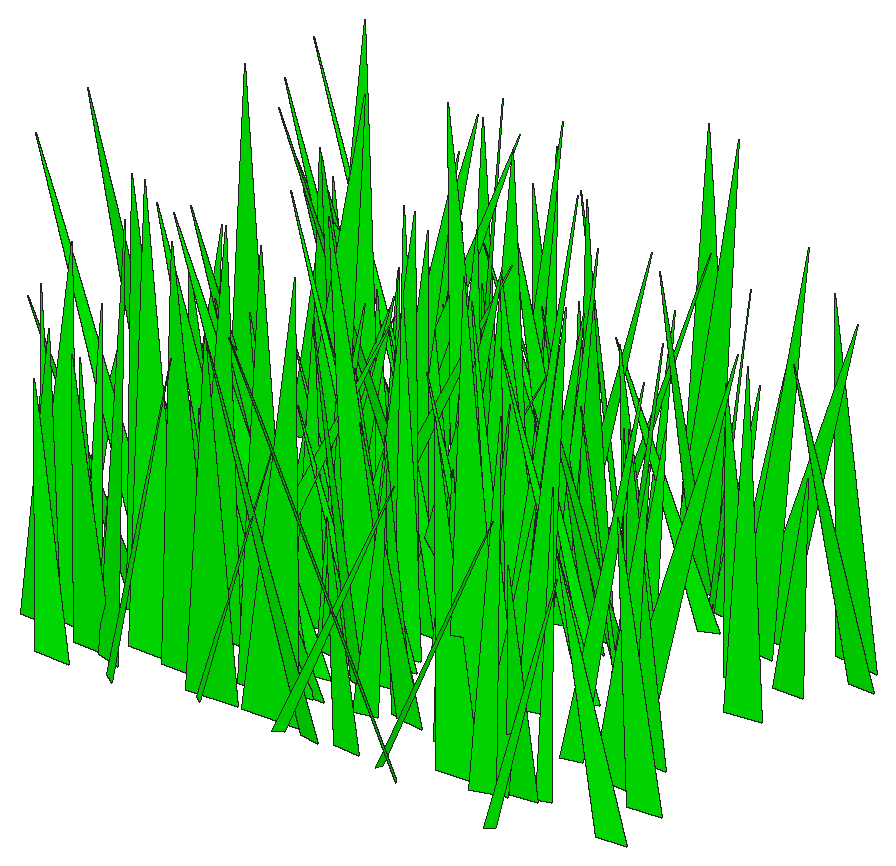
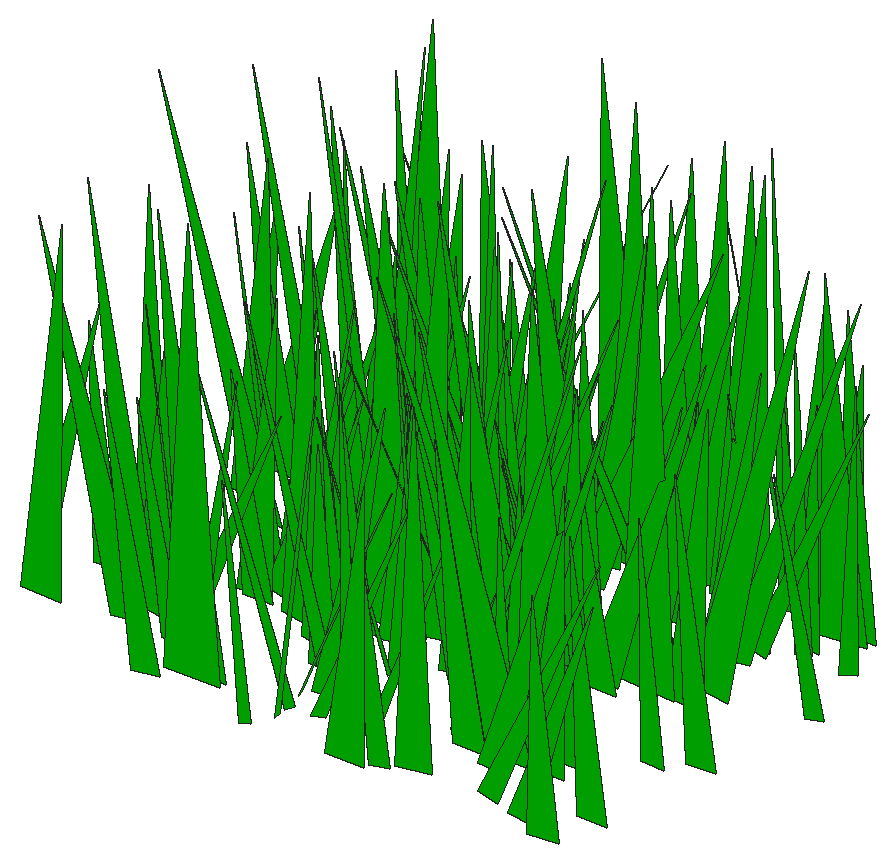
# SketchUp Ruby script. Lengths in inches.
U = 1.inch
M = Sketchup.active_model
def pt(a) = Geom::Point3d.new(a.map { |v| v * U })
def face(e, loops, mat)
  f = e.add_face(loops[0].map { |a| pt(a) })
  loops[1..].each { |l| e.add_face(l.map { |a| pt(a) }).erase! }
  f.material = f.back_material = mat if mat
  f
end
# faces: each face lists its corners as indices into pts; further lists are holes
def faces(e, pts, list, mat = nil) = list.each { |f| face(e, (f[0].is_a?(Array) ? f : [f]).map { |l| l.map { |i| pts[i] } }, mat) }
# xy, xz, yz: faces in a plane at the given z, y or x. An outline is a flat list of corners, or four numbers for a rectangle; further outlines are holes
def ring(l) = l.size == 4 ? [[l[0], l[1]], [l[2], l[1]], [l[2], l[3]], [l[0], l[3]]] : l.each_slice(2).to_a
def flat(e, list, mat, &to3) = list.each { |f| face(e, (f[0].is_a?(Array) ? f : [f]).map { |l| ring(l).map { |u, v| to3.(u, v) } }, mat) }
def xy(e, z, list, mat = nil) = flat(e, list, mat) { |x, y| [x, y, z] }
def xz(e, y, list, mat = nil) = flat(e, list, mat) { |x, z| [x, y, z] }
def yz(e, x, list, mat = nil) = flat(e, list, mat) { |y, z| [x, y, z] }
def lines(e, pts, list) = list.each { |a, b| e.add_line(pt(pts[a]), pt(pts[b])) }
# prism: a flat outline (further loops are holes) pulled along v
def prism(e, loops, v, mat = nil)
  f = face(e, loops, mat); d = Geom::Vector3d.new(v.map { |x| x * U })
  f.pushpull(f.normal.samedirection?(d) ? d.length : -d.length)
end
def box(e, o, s, mat = nil) = prism(e, [[o, [o[0] + s[0], o[1], o[2]], [o[0] + s[0], o[1] + s[1], o[2]], [o[0], o[1] + s[1], o[2]]]], [0, 0, s[2]], mat)
def at(x, y, z, deg = 0) = Geom::Transformation.translation(pt([x, y, z])) * Geom::Transformation.rotation(ORIGIN, Z_AXIS, deg.degrees)
def axes(o, x, y, z) = Geom::Transformation.new([*x, 0, *y, 0, *z, 0, *pt(o).to_a, 1])
def part(name) = M.definitions.add(name)
# library, detail: a bought-in or finely detailed component or shape, given as its bounding box
def library(name, o, s) = part(name).tap { |d| box(d.entities, o, s) }
def detail(e, o, s) = box(e.add_group.entities, o, s)
def put(e, d, t, mat = nil) = e.add_instance(d, t).tap { |i| i.material = mat if mat }
def group(e, t, mat = nil) = e.add_group.tap { |g| g.transformation = t; g.material = mat if mat }.entities
root = M.entities
M.materials.add("[0065_Lime]").color = [0, 255, 0]
c1 = part("fur_instance\#9")
p = [[0.8125,0,1.79],[0.67,-0.02,1.48],[0,-0.11,0],[0,0.11,0]]
faces(c1.entities,p,[[0,1,2,3]])
put(root,c1,axes([47.23,21.45,1.48],[4.4292,-0.25222,2.09729],[2.23078,0.69345,-0.32267],[-2.2121,0.1943,3.87394]),"[0065_Lime]")
put(root,c1,axes([46.43,23.84,1.48],[3.37907,-0.32218,0.93432],[2.44204,0.48577,-0.23052],[-0.78289,0.12464,3.31359]),"[0065_Lime]")
put(root,c1,axes([47.11,27.62,1.48],[2.95,-0.56759,1.1379],[4.20157,0.42898,-0.03681],[-0.78709,0.16263,4.06838]),"[0065_Lime]")
put(root,c1,axes([49.87,22.73,1.48],[-7.12168,0.44148,0.88746],[-3.20755,-1.0075,-0.23593],[0.8793,-0.09949,6.32715]),"[0065_Lime]")
put(root,c1,axes([49.4,24.42,1.48],[-5.61424,-0.877,1.17279],[6.33943,-0.79934,0.04951],[0.91831,0.15643,6.82825]),"[0065_Lime]")
put(root,c1,axes([49.0625,32.54,1.48],[-2.29448,-0.55155,0.20796],[3.93163,-0.32033,0.23303],[-0.11894,0.0513,3.69087]),"[0065_Lime]")
put(root,c1,axes([48,32.97,1.48],[-0.85767,0.65446,0.46875],[-4.67473,-0.1264,0.25449],[0.4141,-0.07144,3.84377]),"[0065_Lime]")
put(root,c1,axes([49.78,22,1.48],[-4.29564,-0.46868,0.1591],[3.34086,-0.60308,0.15104],[0.04046,0.03747,4.42116]),"[0065_Lime]")
put(root,c1,axes([47.57,31.5,1.48],[2.89563,-0.58713,0.52134],[4.16251,0.41505,0.36618],[-0.73658,0.03742,4.11881]),"[0065_Lime]")
put(root,c1,axes([48.19,28.26,1.48],[-2.15247,-0.46889,1.6236],[3.6972,-0.34608,-0.10604],[1.204,0.22446,3.22823]),"[0065_Lime]")
put(root,c1,axes([48.4,20.17,1.48],[-1.17696,0.95171,1.12358],[-6.87953,-0.18043,0.35304],[0.67218,-0.1802,5.58054]),"[0065_Lime]")
put(root,c1,axes([48.27,19.83,1.48],[0.67146,-0.84255,0.3532],[6.0109,0.09305,-0.12296],[0.10231,0.06299,4.90622]),"[0065_Lime]")
put(root,c1,axes([50.43,32.16,1.48],[-4.06579,-0.47447,0.17632],[3.38281,-0.56903,0.30067],[-0.07001,0.0594,4.28842]),"[0065_Lime]")
put(root,c1,axes([48.91,21.03,1.48],[-2.22554,-0.48819,1.56603],[3.88886,-0.33093,0.19972],[0.80849,0.24793,3.35014]),"[0065_Lime]")
put(root,c1,axes([48.77,21.35,1.48],[4.78206,-0.26753,1.75717],[2.0609,0.72896,0.00803],[-2.01098,0.11088,4.18673]),"[0065_Lime]")
put(root,c1,axes([49.67,18.54,1.48],[-1.89741,0.6773,0.01247],[-4.81189,-0.2663,0.24042],[0.28063,0.01321,4.20666]),"[0065_Lime]")
put(root,c1,axes([49.51,25.29,1.48],[-0.06571,-0.77818,0.68187],[5.59689,-0.00459,0.18134],[-0.21553,0.11807,4.50131]),"[0065_Lime]")
put(root,c1,axes([49.87,23.66,1.48],[-2.57835,-0.75231,0.50608],[5.36351,-0.3677,-0.23597],[0.53244,0.06089,4.82782]),"[0065_Lime]")
put(root,c1,axes([50.07,30.28,1.48],[-1.31314,0.71883,1.28918],[-5.35298,-0.18318,-0.18498],[0.16371,-0.22381,4.29201]),"[0065_Lime]")
put(root,c1,axes([51.72,29.89,1.48],[-6.71262,0.39548,0.95592],[-2.87689,-0.95358,-0.14683],[1.01275,-0.08753,5.91881]),"[0065_Lime]")
put(root,c1,axes([49.99,29.61,1.48],[-0.14768,-1.00225,0.25056],[7.13724,-0.02175,-0.13172],[0.16842,0.04279,5.80148]),"[0065_Lime]")
put(root,c1,axes([50.23,19.51,1.48],[-0.42754,-0.82229,0.31765],[5.8646,-0.06048,-0.02331],[0.0571,0.05443,4.77261]),"[0065_Lime]")
put(root,c1,axes([51.22,30.94,1.48],[-2.63269,-0.7093,0.04104],[5.0473,-0.37,-0.05484],[0.08311,0.0019,4.63047]),"[0065_Lime]")
put(root,c1,axes([50.49,21.79,1.48],[0.80245,-1.23017,0.66425],[8.78031,0.11819,0.31677],[-0.46395,0.10914,7.1439]),"[0065_Lime]")
put(root,c1,axes([51.98,25.59,1.48],[-4.04821,-0.74608,0.44801],[5.33652,-0.56795,0.21143],[0.12629,0.08372,5.42684]),"[0065_Lime]")
put(root,c1,axes([50.375,19.72,1.48],[3.47743,-0.24304,1.39652],[2.02024,0.52259,-0.28083],[-1.36303,0.15451,3.14665]),"[0065_Lime]")
put(root,c1,axes([50.79,25.26,1.48],[-2.93002,-1.1104,3.08242],[8.67927,-0.44549,0.08108],[1.21487,0.50458,6.85493]),"[0065_Lime]")
put(root,c1,axes([50.83,29.24,1.48],[-0.74135,1.30052,0.49003],[-9.27229,-0.1059,0.13632],[0.21549,-0.08248,7.55119]),"[0065_Lime]")
put(root,c1,axes([50.4,21.22,1.48],[2.7644,0.47656,0.67631],[-3.38313,0.40243,-0.35262],[-0.86477,-0.05094,3.54148]),"[0065_Lime]")
put(root,c1,axes([52.57,22.97,1.48],[-5.0713,0.71122,0.87309],[-5.15149,-0.71375,-0.31492],[0.48207,-0.14533,5.81953]),"[0065_Lime]")
put(root,c1,axes([51.93,24.83,1.48],[-1.94658,-0.68112,0.62782],[4.90798,-0.26876,0.29807],[-0.05682,0.11979,4.23839]),"[0065_Lime]")
put(root,c1,axes([50.88,19.33,1.48],[-6.55389,-0.45489,2.97592],[3.6482,-1.02785,0.05119],[3.24894,0.23653,5.94567]),"[0065_Lime]")
put(root,c1,axes([53.26,29.8125,1.48],[-8.14536,0.22202,1.03626],[-1.53362,-1.15823,0.33952],[1.32949,0.02421,6.7405]),"[0065_Lime]")
put(root,c1,axes([51.75,20.25,1.48],[-2.01765,1.17085,1.09515],[-8.43103,-0.28877,0.06798],[0.39907,-0.18107,6.97322]),"[0065_Lime]")
put(root,c1,axes([50.26,28.41,1.48],[3.82268,0.39815,0.44658],[-2.87134,0.53759,0.20153],[-0.29195,-0.07403,3.8652]),"[0065_Lime]")
put(root,c1,axes([51.46,30.24,1.48],[-2.79502,0.37495,1.5795],[-3.00222,-0.43736,-0.03599],[1.37024,-0.19344,3.14302]),"[0065_Lime]")
put(root,c1,axes([52.24,27.98,1.48],[-1.87166,-1.01335,0.70925],[7.25339,-0.26757,-0.14548],[0.39328,0.1122,6.05855]),"[0065_Lime]")
put(root,c1,axes([52.27,21.88,1.48],[3.18095,-0.24835,1.55497],[1.95904,0.50766,0.06543],[-1.71476,0.11928,2.95928]),"[0065_Lime]")
put(root,c1,axes([54.47,28.02,1.48],[-7.29785,-0.48829,0.51769],[3.46077,-1.02937,-0.2554],[0.7096,-0.00154,6.56981]),"[0065_Lime]")
put(root,c1,axes([51.38,28.3125,1.48],[-2.54827,-0.40995,2.16007],[3.3881,-0.45499,-0.24896],[2.02097,0.24586,3.14103]),"[0065_Lime]")
put(root,c1,axes([51.65,27.09,1.48],[3.53407,0.45813,0.7792],[-3.26627,0.51155,-0.27665],[-0.93747,-0.05523,3.90131]),"[0065_Lime]")
put(root,c1,axes([52.64,28.46,1.48],[3.40763,-0.27593,1.90182],[2.47601,0.5378,-0.32072],[-1.78658,0.21906,3.18296]),"[0065_Lime]")
put(root,c1,axes([51.17,30.375,1.48],[3.15132,0.98904,0.84715],[-7.11513,0.4384,0.36136],[-0.01573,-0.15909,6.26244]),"[0065_Lime]")
put(root,c1,axes([52.25,22.07,1.48],[1.96154,0.9156,2.8317],[-7.35658,0.28841,0.24682],[-0.67613,-0.48175,5.52958]),"[0065_Lime]")
put(root,c1,axes([51.5,18.59,1.48],[5.99318,0.19121,1.37292],[-1.45464,0.87161,0.13377],[-1.60761,-0.07586,4.99721]),"[0065_Lime]")
put(root,c1,axes([52.79,32.27,1.48],[-4.08034,0.68378,1.87075],[-5.08436,-0.62274,0.28991],[1.76586,-0.21302,5.15743]),"[0065_Lime]")
put(root,c1,axes([52.1,26.04,1.48],[2.00461,1.23257,1.45558],[-8.95105,0.28033,0.2018],[-0.15193,-0.25296,7.31616]),"[0065_Lime]")
put(root,c1,axes([52.97,20.05,1.48],[-0.12204,-1.13464,1.32187],[8.23646,-0.0155,0.05733],[-0.04733,0.22847,6.56856]),"[0065_Lime]")
put(root,c1,axes([52.37,30.51,1.48],[1.80119,0.69196,1.38518],[-5.20498,0.25057,0.28386],[-0.23909,-0.24194,4.2556]),"[0065_Lime]")
put(root,c1,axes([55.44,21.94,1.48],[-6.13954,0.70094,0.10061],[-4.98964,-0.86263,-0.07578],[0.03724,-0.02112,6.43408]),"[0065_Lime]")
put(root,c1,axes([54.4,25.27,1.48],[-4.60606,0.01384,0.73954],[-0.16863,-0.65763,-0.2825],[0.89882,-0.05246,3.73682]),"[0065_Lime]")
put(root,c1,axes([51.26,29.71,1.48],[6.63129,0.66177,0.71913],[-4.76645,0.93275,0.31877],[-0.49172,-0.11701,6.60818]),"[0065_Lime]")
put(root,c1,axes([53.15,31.33,1.48],[7.30412,-0.01994,2.19479],[0.0411,1.09352,0.24234],[-2.70166,-0.03726,5.93745]),"[0065_Lime]")
put(root,c1,axes([53.78,23.91,1.48],[3.70468,-0.58018,1.44831],[4.23681,0.55898,0.33298],[-1.50587,0.14537,4.49994]),"[0065_Lime]")
put(root,c1,axes([54.49,32.97,1.48],[-1.3105,0.78874,0.29597],[-5.6249,-0.18366,-0.07831],[-0.01122,-0.05287,4.68793]),"[0065_Lime]")
put(root,c1,axes([55.26,30.56,1.48],[-3.69418,-0.23516,0.4105],[1.71348,-0.51995,0.22151],[0.34542,0.06432,3.2914]),"[0065_Lime]")
put(root,c1,axes([53.58,32.66,1.48],[6.56596,-0.3231,1.71503],[2.333,0.96687,0.19409],[-2.07118,0.0648,5.65553]),"[0065_Lime]")
put(root,c1,axes([54.17,19.44,1.48],[1.31811,-1.07028,0.00043],[7.60972,0.18505,0.26911],[-0.32609,-0.00785,6.28185]),"[0065_Lime]")
put(root,c1,axes([53.68,25.57,1.48],[2.35032,0.47932,0.58753],[-3.48355,0.32803,0.25266],[-0.14903,-0.10848,3.36001]),"[0065_Lime]")
put(root,c1,axes([53.28,27.46,1.48],[6.49266,-0.71764,1.52624],[5.25924,0.93295,-0.10336],[-1.39403,0.17738,6.71846]),"[0065_Lime]")
put(root,c1,axes([54.53,32.6,1.48],[5.73438,-0.26141,2.21074],[2.2169,0.87344,-0.3438],[-2.43578,0.17953,4.89168]),"[0065_Lime]")
put(root,c1,axes([52.2,22.8,1.48],[6.30052,0.49234,0.17348],[-3.50968,0.88467,0.20459],[-0.06398,-0.04546,5.86051]),"[0065_Lime]")
put(root,c1,axes([55.14,27.64,1.48],[-4.02548,0.57884,1.30914],[-4.18319,-0.59759,0.34327],[1.43523,-0.11828,4.67236]),"[0065_Lime]")
put(root,c1,axes([56.44,31.6,1.48],[-4.74214,0.23885,0.25626],[-1.69737,-0.66782,0.07541],[0.32786,-0.00265,4.09694]),"[0065_Lime]")
put(root,c1,axes([55.69,20.93,1.48],[-4.58117,0.66209,1.03081],[-4.75356,-0.66072,0.24269],[1.10036,-0.09778,5.34006]),"[0065_Lime]")
put(root,c1,axes([54.57,26.84,1.48],[0.12519,0.90816,1.54224],[-6.73073,0.00704,0.22252],[0.24835,-0.26691,5.25331]),"[0065_Lime]")
put(root,c1,axes([55.18,24.41,1.48],[-3.13246,0.48304,0.9905],[-3.46535,-0.46453,0.33998],[1.13621,-0.08507,3.76765]),"[0065_Lime]")
put(root,c1,axes([54.83,23.56,1.48],[2.42727,-0.58743,1.01618],[4.27025,0.36107,0.24531],[-0.89544,0.12954,3.9244]),"[0065_Lime]")
put(root,c1,axes([56.2,21.03,1.48],[-2.4252,-0.49908,0.18297],[3.55594,-0.33828,0.26587],[-0.14382,0.05196,3.48816]),"[0065_Lime]")
put(root,c1,axes([53.95,19.16,1.48],[5.0056,0.1335,0.79462],[-0.96794,0.71617,0.00241],[-0.9592,-0.02601,4.14431]),"[0065_Lime]")
put(root,c1,axes([55.13,20.45,1.48],[-0.75065,-1.13661,1.87157],[8.39979,-0.11704,-0.15281],[0.40697,0.31931,6.606]),"[0065_Lime]")
put(root,c1,axes([56.58,22.91,1.48],[-4.12783,0.24962,0.61548],[-1.85509,-0.58231,-0.31794],[0.53571,-0.09303,3.64151]),"[0065_Lime]")
put(root,c1,axes([54.625,28.02,1.48],[3.10545,0.5802,0.72513],[-4.18816,0.44317,-0.01474],[-0.55054,-0.09856,4.20248]),"[0065_Lime]")
put(root,c1,axes([55.38,23.04,1.48],[-1.76012,-0.65762,1.78715],[5.0861,-0.27878,-0.12322],[0.92795,0.28065,4.06522]),"[0065_Lime]")
put(root,c1,axes([57.03,23.62,1.48],[-4.37671,0.58013,0.55057],[-4.16274,-0.61761,-0.08801],[0.41758,-0.07638,4.89324]),"[0065_Lime]")
put(root,c1,axes([57.63,23.08,1.48],[-8.16969,0.19733,1.17611],[-1.34853,-1.16551,0.35474],[1.49801,0.02694,6.73345]),"[0065_Lime]")
put(root,c1,axes([57.46,19.31,1.48],[-5.96996,-0.449,0.97046],[3.29159,-0.84699,0.26596],[0.89398,0.12015,5.50145]),"[0065_Lime]")
put(root,c1,axes([56.87,30.63,1.48],[-3.63253,0.64668,0.93106],[-4.7153,-0.51413,-0.20621],[0.50577,-0.14862,4.76459]),"[0065_Lime]")
put(root,c1,axes([53.13,26.32,1.48],[7.25901,-0.32559,0.26107],[2.32884,1.01973,-0.22824],[-0.22015,0.0513,6.19388]),"[0065_Lime]")
put(root,c1,axes([56.66,22.29,1.48],[-5.5855,-0.37084,1.47546],[2.64957,-0.82297,-0.29467],[1.79854,0.06073,5.01627]),"[0065_Lime]")
put(root,c1,axes([57.53,30.96,1.48],[-4.58838,-0.01997,0.33202],[0.1625,-0.64643,0.18288],[0.4005,0.03348,3.72956]),"[0065_Lime]")
put(root,c1,axes([56.16,28.53,1.48],[-3.20737,-0.60107,1.34124],[4.39299,-0.48382,-0.31489],[1.31071,0.15074,4.33747]),"[0065_Lime]")
put(root,c1,axes([55.98,24.45,1.48],[-6.19842,0.14888,2.41809],[-1.09563,-0.96491,0.13257],[2.95966,-0.04539,5.11329]),"[0065_Lime]")
put(root,c1,axes([57.03,22.62,1.48],[-3.80468,0.96953,1.86173],[-7.23157,-0.54178,-0.32383],[0.74076,-0.30941,6.40083]),"[0065_Lime]")
put(root,c1,axes([57.16,25.25,1.48],[-4.92857,0.27745,1.14097],[-2.10496,-0.71174,-0.21653],[1.19806,-0.10912,4.31329]),"[0065_Lime]")
put(root,c1,axes([57.02,26.66,1.48],[-6.50986,0.84997,2.24696],[-6.23212,-0.9693,0.34024],[2.31956,-0.21884,7.22025]),"[0065_Lime]")
put(root,c1,axes([56.01,19.54,1.48],[2.78966,-1.11729,1.54568],[8.15235,0.40126,-0.01582],[-0.61028,0.25289,6.85414]),"[0065_Lime]")
put(root,c1,axes([57.28,32.21,1.48],[-5.8952,0.0148,1.57894],[-0.00586,-0.87111,0.25906],[1.94397,0.04224,4.789]),"[0065_Lime]")
put(root,c1,axes([56.15,24.26,1.48],[0.8068,-1.11162,2.12559],[8.32936,0.09956,-0.34711],[0.18211,0.37118,6.45891]),"[0065_Lime]")
put(root,c1,axes([56.83,24.125,1.48],[-7.03207,0.38953,2.81846],[-3.12357,-1.08256,-0.14293],[3.15179,-0.20378,6.14671]),"[0065_Lime]")
put(root,c1,axes([54.82,27.12,1.48],[5.19461,0.15153,0.00889],[-1.07445,0.72784,-0.32831],[-0.09271,0.05522,4.30294]),"[0065_Lime]")
put(root,c1,axes([57.5,27.39,1.48],[3.13497,-0.29778,1.79348],[2.47434,0.50773,-0.03679],[-1.79723,0.17959,3.07777]),"[0065_Lime]")
put(root,c1,axes([57.36,25.82,1.48],[1.2554,0.60019,0.55742],[-4.30563,0.18305,-0.18872],[-0.4182,-0.08296,3.61634]),"[0065_Lime]")
put(root,c1,axes([56.36,28.78,1.48],[4.30443,0.00922,0.50487],[-0.09222,0.61051,0.14652],[-0.61729,-0.0269,3.49862]),"[0065_Lime]")
put(root,c1,axes([57.78,26.77,1.48],[-0.80012,1.27765,0.34789],[-9.10112,-0.11333,0.09778],[0.15737,-0.05838,7.42384]),"[0065_Lime]")
put(root,c1,axes([56.26,25.39,1.48],[4.80138,-0.81518,1.06965],[5.92306,0.6771,-0.29996],[-0.54904,0.17572,6.11804]),"[0065_Lime]")
put(root,c1,axes([60.54,19,1.48],[-7.40306,-0.12302,0.2961],[0.89245,-1.04008,0.28396],[0.32006,0.05477,6.05705]),"[0065_Lime]")
put(root,c1,axes([57.89,29.58,1.48],[0.57177,0.61134,0.45851],[-4.37536,0.08528,-0.20017],[-0.31933,-0.07387,3.56367]),"[0065_Lime]")
put(root,c1,axes([57.94,24.86,1.48],[-0.25077,1.17206,0.00642],[-8.34102,-0.03524,0.00696],[0.00879,-0.00107,6.78776]),"[0065_Lime]")
put(root,c1,axes([57.68,33.05,1.48],[3.88302,-0.16494,1.16701],[1.27106,0.57753,-0.063],[-1.34931,0.06938,3.29906]),"[0065_Lime]")
put(root,c1,axes([57.79,21.2,1.48],[3.58678,-0.45362,1.16886],[3.3351,0.52966,0.1166],[-1.16767,0.1194,3.92347]),"[0065_Lime]")
put(root,c1,axes([58.95,21.53,1.48],[-3.38913,-0.56186,0.98202],[4.11078,-0.48738,0.04263],[0.73954,0.13429,4.26335]),"[0065_Lime]")
put(root,c1,axes([58.55,19.47,1.48],[-1.75927,-0.52415,0.86248],[3.84246,-0.25768,-0.0616],[0.52295,0.13005,3.35408]),"[0065_Lime]")
put(root,c1,axes([58.69,21.59,1.48],[-3.39932,-0.49232,1.37448],[3.67426,-0.50991,-0.10775],[1.27683,0.15664,3.96934]),"[0065_Lime]")
put(root,c1,axes([56.59,19.15,1.48],[5.55039,-0.18622,0.31887],[1.33416,0.78147,-0.07289],[-0.36039,0.02507,4.64109]),"[0065_Lime]")
put(root,c1,axes([57.43,29.96,1.48],[5.70138,0.45009,0.99033],[-3.21366,0.81758,-0.20993],[-1.18922,-0.05157,5.31518]),"[0065_Lime]")
put(root,c1,axes([59.44,25.8125,1.48],[-2.78019,0.91541,0.55709],[-6.53239,-0.39521,0.19114],[0.48581,-0.07544,5.75821]),"[0065_Lime]")
put(root,c1,axes([58.86,28.66,1.48],[3.02424,0.61197,1.71769],[-4.61478,0.47009,-0.23625],[-1.45946,-0.21831,4.30637]),"[0065_Lime]")
put(root,c1,axes([57.27,31.72,1.48],[6.28974,-0.10629,0.83186],[0.81876,0.89311,-0.27216],[-0.97347,0.06442,5.14583]),"[0065_Lime]")
put(root,c1,axes([60.15,23.61,1.48],[-5.07099,0.32937,0.99573],[-2.45019,-0.72516,-0.21833],[0.99461,-0.10714,4.53889]),"[0065_Lime]")
put(root,c1,axes([58.64,27.95,1.48],[6.63672,-0.22192,1.91623],[1.72592,0.98446,-0.13468],[-2.25057,0.10056,5.5475]),"[0065_Lime]")
put(root,c1,axes([58.39,27.41,1.48],[5.01943,-0.55593,0.9728],[3.94487,0.72327,0.38294],[-1.23319,0.05089,5.18455]),"[0065_Lime]")
put(root,c1,axes([60.27,27.51,1.48],[-5.07243,-0.40044,1.29073],[2.95805,-0.73846,0.01438],[1.37444,0.11146,4.73253]),"[0065_Lime]")
put(root,c1,axes([59.53,22.58,1.48],[0.40661,0.59501,1.11937],[-4.44628,0.06443,-0.079],[-0.23312,-0.19107,3.45924]),"[0065_Lime]")
put(root,c1,axes([60.5,27.03,1.48],[-3.81655,0.25552,0.55947],[-1.83982,-0.54351,0.01373],[0.62828,-0.0394,3.43876]),"[0065_Lime]")
put(root,c1,axes([60.41,23.375,1.48],[-2.51475,-0.47159,0.63145],[3.42716,-0.35614,0.11766],[0.34749,0.09964,3.40922]),"[0065_Lime]")
put(root,c1,axes([59.88,28,1.48],[-4.53459,-0.78813,2.72613],[6.26195,-0.68786,0.228],[1.86514,0.39325,5.86235]),"[0065_Lime]")
put(root,c1,axes([60.53,31.59,1.48],[-4.58749,-0.37891,1.41998],[2.9439,-0.66704,0.32839],[1.28533,0.17542,4.31594]),"[0065_Lime]")
put(root,c1,axes([58.86,25.69,1.48],[8.58228,-0.20651,2.16498],[1.57121,1.2601,-0.09344],[-2.60292,0.07976,7.08193]),"[0065_Lime]")
put(root,c1,axes([61.35,27.22,1.48],[-3.63898,-0.41173,0.58788],[3.00017,-0.51077,0.30051],[0.3267,0.10441,3.78837]),"[0065_Lime]")
put(root,c1,axes([59.77,23.49,1.48],[4.83063,0.32559,1.67082],[-2.61356,0.71554,0.32723],[-1.66049,-0.17906,4.34562]),"[0065_Lime]")
put(root,c1,axes([60.24,32.01,1.48],[-0.81872,1.09987,2.35055],[-8.33524,-0.12615,0.05713],[0.37503,-0.40275,6.40129]),"[0065_Lime]")
put(root,c1,axes([61.94,30.05,1.48],[-4.08184,0.39913,0.20903],[-2.85157,-0.57226,-0.22776],[0.05045,-0.05293,4.03858]),"[0065_Lime]")
put(root,c1,axes([60.41,21.16,1.48],[2.87807,0.42087,1.75164],[-3.44183,0.44446,0.16322],[-1.32735,-0.23994,3.37481]),"[0065_Lime]")
put(root,c1,axes([61.96,25.2,1.48],[-5.57645,0.29413,0.84583],[-2.17606,-0.79132,-0.27135],[0.853,-0.09582,4.83738]),"[0065_Lime]")
put(root,c1,axes([60.13,31.69,1.48],[4.30665,0.97668,1.74722],[-7.15841,0.63144,-0.15329],[-1.29669,-0.24208,6.64923]),"[0065_Lime]")
put(root,c1,axes([61.66,20.17,1.48],[-1.14449,0.9193,0.15698],[-6.5415,-0.15975,-0.20632],[-0.21673,-0.03284,5.39842]),"[0065_Lime]")
put(root,c1,axes([61.73,27.59,1.48],[-3.09016,0.63704,1.27299],[-4.70934,-0.45255,0.02507],[0.90791,-0.17917,4.46275]),"[0065_Lime]")
put(root,c1,axes([62.05,26.2,1.48],[-4.77578,-0.00643,1.22138],[-0.00021,-0.70317,-0.12453],[1.50225,-0.02053,3.88286]),"[0065_Lime]")
put(root,c1,axes([60.98,23.98,1.48],[5.9272,-0.63589,1.88493],[4.69018,0.87693,0.15491],[-1.96228,0.17526,6.06382]),"[0065_Lime]")
put(root,c1,axes([59.75,19.32,1.48],[5.66233,-0.07479,0.34698],[0.51574,0.79744,0.19148],[-0.44643,-0.02742,4.62216]),"[0065_Lime]")
put(root,c1,axes([62.21,20.25,1.48],[-1.63123,1.2715,0.87046],[-9.11041,-0.23023,-0.02686],[0.15714,-0.14882,7.47893]),"[0065_Lime]")
put(root,c1,axes([61.47,27.79,1.48],[0.2524,0.63001,0.24286],[-4.49018,0.03377,0.15209],[0.17033,-0.04333,3.64953]),"[0065_Lime]")
put(root,c1,axes([61.3,30.96,1.48],[5.66071,0.2108,1.52948],[-1.44747,0.8381,-0.3261],[-1.92118,-0.01033,4.75227]),"[0065_Lime]")
put(root,c1,axes([62.02,26.64,1.48],[4.1716,-0.15053,1.54257],[1.02241,0.64372,0.27547],[-1.92317,0.01571,3.49248]),"[0065_Lime]")
put(root,c1,axes([62.71,21.05,1.48],[-7.59138,0.33554,2.15426],[-2.40525,-1.12802,0.27942],[2.63266,-0.06303,6.46717]),"[0065_Lime]")
put(root,c1,axes([61.3,32.59,1.48],[2.73112,-0.54597,1.00785],[4.05642,0.3853,-0.27891],[-0.42075,0.1707,3.85302]),"[0065_Lime]")
put(root,c1,axes([61.71,30.91,1.48],[2.52874,0.51762,0.58375],[-3.70372,0.36383,-0.19475],[-0.60549,-0.06373,3.62917]),"[0065_Lime]")
put(root,c1,axes([61.62,26.66,1.48],[5.87374,0.27865,1.56874],[-2.06114,0.86508,-0.04282],[-1.84484,-0.07934,5.04252]),"[0065_Lime]")
put(root,c1,axes([62.63,19.92,1.48],[5.81615,-0.45904,1.98053],[3.39729,0.87558,0.19922],[-2.24915,0.13549,5.42244]),"[0065_Lime]")
put(root,c1,axes([62.73,20.125,1.48],[1.85592,0.73816,0.62888],[-5.3062,0.26202,0.0551],[-0.19305,-0.10563,4.53146]),"[0065_Lime]")
put(root,c1,axes([63.61,20.33,1.48],[0.95982,-0.6406,0.27831],[4.54486,0.13902,0.35164],[-0.49436,0.03429,3.77317]),"[0065_Lime]")
put(root,c1,axes([64.22,28.52,1.48],[0.5241,0.71238,1.2867],[-5.27608,0.09532,-0.34647],[-0.60571,-0.21388,4.13122]),"[0065_Lime]")
put(root,c1,axes([63.51,29.9375,1.48],[4.87832,0.82116,1.41667],[-5.93667,0.71115,-0.28686],[-1.39263,-0.15509,6.18536]),"[0065_Lime]")
put(root,c1,axes([64.15,20.55,1.48],[-4.98897,0.23107,1.97762],[-1.69867,-0.77674,0.2059],[2.3937,-0.0696,4.2679]),"[0065_Lime]")
put(root,c1,axes([63.37,22.65,1.48],[6.85913,-0.33502,1.65008],[2.56798,0.99482,-0.29461],[-1.79028,0.14339,5.8994]),"[0065_Lime]")
put(root,c1,axes([64.92,23.6875,1.48],[-0.10352,-0.85695,1.18163],[6.2685,-0.01118,0.09158],[-0.09107,0.20434,4.9605]),"[0065_Lime]")
put(root,c1,axes([63.38,30.65,1.48],[4.73198,-0.69221,0.73484],[4.99592,0.66467,-0.30554],[-0.35163,0.12829,5.54777]),"[0065_Lime]")
put(root,c1,axes([63.94,18.6,1.48],[4.94653,-0.17044,0.82412],[1.23214,0.70884,0.01922],[-0.98973,0.03062,4.14273]),"[0065_Lime]")
put(root,c1,axes([64.98,22.31,1.48],[2.00532,0.78999,1.04716],[-5.75459,0.28687,0.03936],[-0.38587,-0.17271,4.85506]),"[0065_Lime]")
put(root,c1,axes([63.92,24.38,1.48],[5.74819,0.75924,0.9259],[-5.45589,0.8165,-0.0245],[-0.85024,-0.10643,6.41693]),"[0065_Lime]")
put(root,c1,axes([65.39,27.13,1.48],[3.56725,-0.68128,1.97869],[5.21552,0.54321,0.04608],[-1.49078,0.27023,4.89595]),"[0065_Lime]")
put(root,c1,axes([65.96,31.04,1.48],[-2.54409,-0.85844,1.51209],[6.3235,-0.37781,-0.14797],[0.88882,0.23084,5.38086]),"[0065_Lime]")
put(root,c1,axes([66.8,19.97,1.48],[-2.61304,0.60899,0.01657],[-4.33395,-0.36717,-0.02011],[-0.01065,-0.00424,4.1164]),"[0065_Lime]")
put(root,c1,axes([66.81,30.2,1.48],[-3.75238,-0.56484,1.03088],[4.18031,-0.52919,0.35158],[0.53791,0.17231,4.45908]),"[0065_Lime]")
put(root,c1,axes([66.52,21.69,1.48],[-1.28955,0.71334,0.51006],[-5.11451,-0.17846,-0.192],[-0.07618,-0.09354,4.2561]),"[0065_Lime]")
put(root,c1,axes([65.49,28.84,1.48],[1.41441,-0.58028,0.47325],[4.16823,0.19947,-0.0467],[-0.13371,0.07997,3.55032]),"[0065_Lime]")
